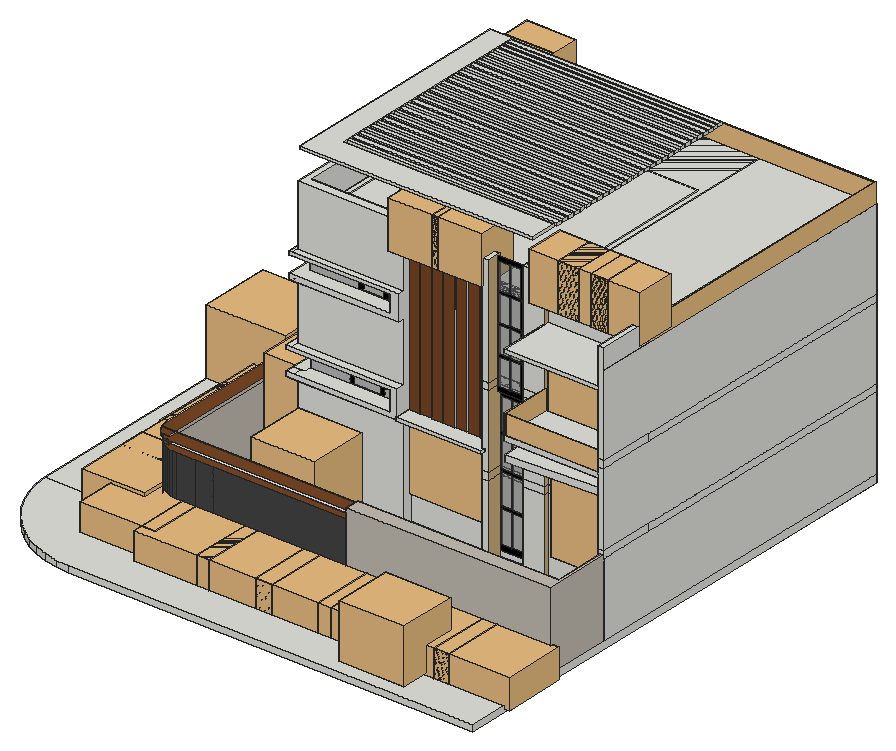
# SketchUp Ruby script. Lengths in inches.
U = 1.inch
M = Sketchup.active_model
def pt(a) = Geom::Point3d.new(a.map { |v| v * U })
def face(e, loops, mat)
  f = e.add_face(loops[0].map { |a| pt(a) })
  loops[1..].each { |l| e.add_face(l.map { |a| pt(a) }).erase! }
  f.material = f.back_material = mat if mat
  f
end
# faces: each face lists its corners as indices into pts; further lists are holes
def faces(e, pts, list, mat = nil) = list.each { |f| face(e, (f[0].is_a?(Array) ? f : [f]).map { |l| l.map { |i| pts[i] } }, mat) }
# xy, xz, yz: faces in a plane at the given z, y or x. An outline is a flat list of corners, or four numbers for a rectangle; further outlines are holes
def ring(l) = l.size == 4 ? [[l[0], l[1]], [l[2], l[1]], [l[2], l[3]], [l[0], l[3]]] : l.each_slice(2).to_a
def flat(e, list, mat, &to3) = list.each { |f| face(e, (f[0].is_a?(Array) ? f : [f]).map { |l| ring(l).map { |u, v| to3.(u, v) } }, mat) }
def xy(e, z, list, mat = nil) = flat(e, list, mat) { |x, y| [x, y, z] }
def xz(e, y, list, mat = nil) = flat(e, list, mat) { |x, z| [x, y, z] }
def yz(e, x, list, mat = nil) = flat(e, list, mat) { |y, z| [x, y, z] }
def lines(e, pts, list) = list.each { |a, b| e.add_line(pt(pts[a]), pt(pts[b])) }
# prism: a flat outline (further loops are holes) pulled along v
def prism(e, loops, v, mat = nil)
  f = face(e, loops, mat); d = Geom::Vector3d.new(v.map { |x| x * U })
  f.pushpull(f.normal.samedirection?(d) ? d.length : -d.length)
end
def box(e, o, s, mat = nil) = prism(e, [[o, [o[0] + s[0], o[1], o[2]], [o[0] + s[0], o[1] + s[1], o[2]], [o[0], o[1] + s[1], o[2]]]], [0, 0, s[2]], mat)
def at(x, y, z, deg = 0) = Geom::Transformation.translation(pt([x, y, z])) * Geom::Transformation.rotation(ORIGIN, Z_AXIS, deg.degrees)
def axes(o, x, y, z) = Geom::Transformation.new([*x, 0, *y, 0, *z, 0, *pt(o).to_a, 1])
def part(name) = M.definitions.add(name)
# library, detail: a bought-in or finely detailed component or shape, given as its bounding box
def library(name, o, s) = part(name).tap { |d| box(d.entities, o, s) }
def detail(e, o, s) = box(e.add_group.entities, o, s)
def put(e, d, t, mat = nil) = e.add_instance(d, t).tap { |i| i.material = mat if mat }
def group(e, t, mat = nil) = e.add_group.tap { |g| g.transformation = t; g.material = mat if mat }.entities
root = M.entities
M.materials.add("[Color D01]").color = [221, 214, 193]
M.materials.add("[Color M00]").color = [255, 255, 255]
M.materials.add("[Color M09]").color = [0, 0, 0]
M.materials.add("[Field Rectangle Tile]").color = [196, 189, 179]
M.materials.add("[Field Rectangle Tile]1").color = [196, 189, 179]
M.materials.add("[Granite Dark Gray]").color = [69, 68, 68]
M.materials.add("[Mirror 01]").color = [185, 185, 185]
M.materials.add("[Translucent_Glass_Gray]").color = [128, 128, 128]
M.materials["[Translucent_Glass_Gray]"].alpha = 0.5
M.materials.add("[Wood Floor Light]").color = [204, 176, 127]
M.materials.add("[Wood Floor]").color = [155, 105, 61]
M.materials.add("[Wood Veneer 01]").color = [120, 70, 37]
c1 = library("window full",[0,0,0],[14.17,66.54,74.02])
c2 = library("PENTEK_RP+Hermetic+70+FP_EI90_Single_Leaf_Door_Top__And_Both",[-0.01,-3.31,-0.39],[86.62,9.05,102.36])
c3 = library("Ver Glass Railing",[0,0,0],[2.5,185,31])
c4 = library("Glazed panel assembly",[0,0,0],[135.86,2.83,115.35])
c5 = part("wndow2")
xz(c5.entities,0,[[[-13,0,13,55],[-11,2,11,53]],[-0.5,2,0.5,2,0.5,14.25,11,14.25,11,15.25,0.5,15.25,0.5,27,11,27,11,28,0.5,28,0.5,39.75,11,39.75,11,40.75,0.5,40.75,0.5,53,-0.5,53,-0.5,40.75,-11,40.75,-11,39.75,-0.5,39.75,-0.5,28,-11,28,-11,27,-0.5,27,-0.5,15.25,-11,15.25,-11,14.25,-0.5,14.25]],"[Color M09]")
xz(c5.entities,0,[[-11,2,-0.5,14.25],[0.5,2,11,14.25],[-11,15.25,-0.5,27],[0.5,15.25,11,27],[-11,28,-0.5,39.75],
  [0.5,28,11,39.75],[-11,40.75,-0.5,53],[0.5,40.75,11,53]],"[Translucent_Glass_Gray]")
c6 = library("windows",[1167.36,374.41,0],[108.46,5.67,65.67])
c7 = library("Round Planter with Plant",[-35.48,-39.77,0],[80.62,63.55,77.875])
c8 = library("GoldenBamboo",[-21.19,-21.7,-0.46],[44.22,41.02,72.81])
c9 = library("Hedge section",[-5.85,-6.78,-4.2],[64.5,123.13,48])
c10 = library("279",[-34.23,-17.84,-5],[65.55,41.78,17.48])
c11 = library("Palm+in+pot",[-44.1,-44.03,0.04],[106.77,95.72,88.04])
c12 = library("ganyedes's+yellow&green+tree",[-30.91,-35.46,0],[63.51,67.02,85.79])
c13 = part("Group\#12")
box(c13.entities,[0,0,0],[344.0625,7.58,4.6875])
xy(root,-12,[[0,161.3125,168.75,829],[265.5625,346.4375,275.875,492.0625],[267.4375,748.89,275.875,808.39]])
xy(root,-10.75,[[275.875,346.4375,438.125,361.3125]])
xy(root,-2.125,[[168.75,0,829.125,0,829.125,161.3125,0,161.3125,2.76,140.16,8.11,119.5,15.95,99.66,26.17,80.9375,38.62,63.61,53.11,47.95,69.41,34.18,87.28,22.53,106.44,13.16,126.62,6.22,147.49,1.81],[0,161.3125,168.75,829]])
xy(root,-1.0625,[[239.8125,808.39,277.27,827.375]])
xy(root,0,[[491.9375,162.5,825.8125,162.5,825.8125,271.3125,819.83,271.3125,819.83,185.9375,491.9375,185.9375],[816.01,271.3125,816.01,361.3125,825.8125,361.3125,825.8125,271.4375,819.83,271.4375,819.83,271.3125],[819.83,271.3125,825.8125,271.4375],[[573.62,338.0625,573.62,361.3125,275.875,361.3125,275.875,827.375,825.8125,827.375,825.8125,361.3125,662.88,361.3125,662.88,353.3125,627,353.3125,627,361.3125,583.89,361.3125,583.89,338.0625],[284.875,370.3125,626.875,712.3125]],[284.875,370.3125,626.875,712.3125],
  [168.75,491.6875,168.75,829,175.75,829,175.75,821.49,195.4375,821.49,195.4375,491.6875],[267.4375,748.89,275.875,808.39],[175.75,821.49,239.8125,829]])
xy(root,0,[[214.63,162.5,208.88,162.86,203.22,163.94,197.73,165.72,192.52,168.17,187.65,171.25,185.98,172.625,194.0625,172.625,194.0625,179.125,491.9375,179.125,491.9375,162.5],[185.98,172.625,183.2,174.92,179.25,179.12,175.85,183.78,173.07,188.82,170.93,194.18,169.49,199.76,168.75,205.47,168.75,491.6875,180.875,491.6875,180.875,179.125,194.0625,179.125,194.0625,172.625]],"[Field Rectangle Tile]")
xy(root,108.91,[[214.63,162.5,491.9375,162.5,491.9375,179.125,194.0625,179.125,194.0625,172.625,185.98,172.625,187.65,171.25,192.52,168.17,197.73,165.72,203.22,163.94,208.88,162.86],[185.98,172.625,194.0625,172.625,194.0625,179.125,180.875,179.125,180.875,491.6875,168.75,491.6875,168.75,205.47,169.49,199.76,170.93,194.18,173.07,188.82,175.85,183.78,179.25,179.12,183.2,174.92]],"[Wood Veneer 01]")
xy(root,118.68,[[206.91,162.5,491.9375,162.5,491.9375,185.9375,195.4375,185.9375,195.4375,171.6875,182.2,171.6875,183.68,170.39,187.83,167.61,192.31,165.41,197.04,163.8,201.93,162.83],[182.2,171.6875,195.4375,171.6875,195.4375,185.9375,171.72,185.9375,173.86,181.58,176.64,177.43,179.93,173.68],[171.72,185.9375,195.4375,185.9375,195.4375,491.6875,168.75,491.6875,168.75,200.66,169.08,195.68,170.05,190.79,171.66,186.06]],"[Wood Veneer 01]")
xy(root,120,[[[816.01,271.3125,819.83,271.3125,819.83,271.4375,825.8125,271.4375,825.8125,827.375,275.875,827.375,275.875,808.39,267.4375,808.39,267.4375,748.89,275.875,748.89,275.875,361.3125,573.62,361.3125,573.62,338.0625,583.89,338.0625,583.89,361.3125,816.01,361.3125],[284.875,370.3125,626.875,712.3125]],[627,353.3125,662.88,361.3125]])
xy(root,120,[[819.83,271.3125,825.8125,271.4375]],"[Field Rectangle Tile]")
xy(root,121.96,[[206.91,162.5,201.93,162.83,197.04,163.8,192.31,165.41,187.83,167.61,183.68,170.39,182.2,171.6875,195.4375,171.6875,195.4375,185.9375,491.9375,185.9375,491.9375,162.5],[182.2,171.6875,179.93,173.68,176.64,177.43,173.86,181.58,171.72,185.9375,195.4375,185.9375,195.4375,171.6875],[171.72,185.9375,171.66,186.06,170.05,190.79,169.08,195.68,168.75,200.66,168.75,491.6875,195.4375,491.6875,195.4375,185.9375]],"[Wood Veneer 01]")
xy(root,124.03,[[175.75,821.49,239.8125,829]],"[Field Rectangle Tile]")
xy(root,125.47,[[491.9375,162.5,491.9375,185.9375,819.83,185.9375,819.83,271.3125,825.8125,271.3125,825.8125,162.5],[168.75,491.6875,195.4375,491.6875,195.4375,821.49,175.75,821.49,175.75,829,168.75,829]],"[Field Rectangle Tile]")
xy(root,132,[[[816.01,271.3125,816.01,361.3125,583.89,361.3125,583.89,338.0625,573.62,338.0625,573.62,361.3125,275.875,361.3125,275.875,748.89,267.4375,748.89,267.4375,808.39,277.27,808.39,277.27,827.375,825.8125,827.375,825.8125,271.3125],[284.875,370.3125,626.875,712.3125]],[627,353.3125,662.88,361.3125],[284.875,370.3125,626.875,712.3125]])
xy(root,160.08,[[438.125,330.8125,438.125,361.3125,573.62,361.3125,573.62,338.0625,577.3125,338.0625,577.3125,330.8125],[573.62,338.0625,577.3125,361.3125]])
xy(root,160.1,[[255.6875,333.625,265.5625,492.0625],[265.5625,333.625,438.125,346.4375]])
xy(root,165.14,[[438.125,330.8125,577.3125,330.8125,577.3125,338.0625,573.62,338.0625,573.62,361.3125,455.875,361.3125,455.875,357.1875,438.125,357.1875],[573.62,338.0625,577.3125,361.3125]])
xy(root,167.29,[[255.6875,333.625,268.5625,349.4375],[268.5625,333.625,425.75,333.625,425.75,361.0625,275.875,361.0625,275.875,349.4375,268.5625,349.4375],[255.6875,349.4375,275.875,478]])
xy(root,199.99,[[255.6875,333.625,268.5625,349.4375],[268.5625,333.625,268.5625,349.4375,275.875,349.4375,275.875,361.0625,425.75,361.0625,425.75,333.625],[255.6875,349.4375,275.875,478]])
xy(root,206.11,[[255.6875,333.625,265.5625,492.0625],[265.5625,333.625,438.125,346.4375]])
xy(root,207.82,[[667.38,267.22,662.88,353.3125,816.01,361.3125,820.5,275.22]])
xy(root,218.69,[[667.38,267.22,820.5,275.22,816.01,361.3125,662.88,353.3125]])
xy(root,225.91,[[223.8125,591.58,275.875,748.89]])
xy(root,232.53,[[223.8125,591.58,275.875,748.89]])
xy(root,235.77,[[662.88,271.3125,816.01,361.3125]])
xy(root,245,[[662.88,271.3125,816.01,361.3125]])
xy(root,252,[[[816.01,271.3125,825.8125,271.3125,825.8125,827.375,239.8125,827.375,239.8125,808.39,267.4375,808.39,267.4375,748.89,275.875,748.89,275.875,361.3125,573.62,361.3125,573.62,338.0625,583.89,338.0625,583.89,361.3125,627,361.3125,627,353.3125,662.88,353.3125,662.88,361.3125,816.01,361.3125],[284.875,370.3125,626.875,712.3125]],[223.8125,591.58,275.875,740.64],[223.8125,740.64,275.875,748.89]])
xy(root,258.25,[[223.8125,601.46,275.875,740.64]])
xy(root,264,[[573.62,337.875,583.89,338.0625],[284.875,370.3125,626.875,712.3125]])
xy(root,302.1875,[[265.5625,336.5625,438.125,346.4375]])
xy(root,302.3,[[259.1875,336.5625,265.5625,492.0625]])
xy(root,310.68,[[259.1875,336.5625,423.3125,336.5625,423.3125,360,274.875,360,274.875,476.5,259.1875,476.5]])
xy(root,337.87,[[268.5625,336.5625,268.5625,349.4375,274.875,349.4375,274.875,360,423.3125,360,423.3125,336.5625]])
xy(root,337.99,[[259.1875,336.5625,259.1875,476.5,274.875,476.5,274.875,349.4375,268.5625,349.4375,268.5625,336.5625]])
xy(root,338.02,[[253.0625,498.98,275.875,565.79]])
xy(root,340.52,[[253.0625,498.98,275.875,565.79]])
xy(root,343.56,[[259.1875,336.5625,265.5625,492.0625],[265.5625,336.5625,438.125,346.4375]])
xy(root,361.8125,[[223.8125,601.46,275.875,740.64]])
xy(root,364.17,[[662.88,271.3125,816.01,361.3125]])
xy(root,369.65,[[662.88,271.3125,816.01,361.3125]])
xy(root,369.9375,[[223.8125,591.58,275.875,743.08],[223.8125,743.08,275.875,748.89]])
xy(root,396,[[825.23,271.3125,825.8125,271.3125,825.8125,827.375,275.875,827.375,275.875,566.29,284.875,566.29,284.875,712.3125,626.875,712.3125,626.875,370.3125,284.875,370.3125,284.875,492.0625,275.875,492.0625,275.875,361.3125,825.23,361.3125],[438.125,357.1875,455.875,361.3125],[457.4375,357.1875,475.1875,361.3125],[476.6875,357.1875,494.4375,361.3125],[496.0625,357.1875,513.8125,361.3125],
  [516.0625,357.1875,533.8125,361.3125],[536.3125,357.1875,554.0625,361.3125],[555.87,357.1875,573.62,361.3125],[409.12,375.75,426.56,383.06],[291.63,576.24,309.26,602.43],
  [293.42,673.58,312.92,704.71]])
xy(root,426.5625,[[275.875,492.0625,284.875,566.29]])
xy(root,428.375,[[816.01,271.3125,825.23,361.3125]])
xy(root,432.4375,[[267.4375,748.89,275.875,827.375],[239.8125,808.39,267.4375,827.375]])
xy(root,443.3125,[[573.62,337.875,583.89,361.3125],[265.5625,346.4375,438.125,346.4375,438.125,361.3125,275.875,361.3125,275.875,492.0625,265.5625,492.0625],[627,353.3125,662.88,361.3125]])
xy(root,493.6875,[[271.05,344.17,271.05,732.64,293.42,732.64,293.42,602.43,291.63,602.43,291.63,576.24,293.42,576.24,293.42,344.17],[293.42,344.17,293.42,576.24,308.57,576.24,308.57,386.78,312.92,386.78,312.92,344.17],[312.92,344.17,312.92,386.78,409.12,386.78,409.12,375.75,426.56,375.75,426.56,386.78,651.74,386.78,651.74,344.17],[409.12,375.75,426.56,383.06],[409.12,383.06,426.56,386.78],
  [291.63,576.24,293.42,602.43],[293.42,576.24,308.57,602.43],[308.57,576.24,309.26,602.43],[293.42,602.43,308.57,673.58],[308.57,673.58,312.92,704.71],
  [293.42,704.71,308.57,732.64]])
xy(root,498.375,[[271.05,344.17,651.74,344.17,651.74,386.78,308.57,386.78,308.57,732.64,271.05,732.64]])
xz(root,0,[[168.75,-12,829.125,-2.125]])
xz(root,161.3125,[[168.75,-12,829.125,-2.125]])
xz(root,162.5,[[206.91,118.68,491.9375,121.96]],"[Color M00]")
xz(root,162.5,[[491.9375,0,825.8125,125.47]],"[Field Rectangle Tile]1")
xz(root,162.5,[[214.63,0,245.35,108.91],[245.35,0,273.69,108.91],[273.69,0,491.9375,108.91]],"[Granite Dark Gray]")
xz(root,171.6875,[[182.2,118.68,195.4375,121.96]],"[Wood Veneer 01]")
xz(root,179.125,[[180.875,0,491.9375,108.91]],"[Field Rectangle Tile]")
xz(root,185.9375,[[491.9375,0,819.83,0,819.83,125.47,491.9375,125.47,491.9375,121.96,171.72,121.96,171.72,118.68,491.9375,118.68]],"[Field Rectangle Tile]")
xz(root,271.3125,[[816.01,0,825.8125,120],[816.01,120,819.83,120,819.83,125.47,825.8125,125.47,825.8125,132,816.01,132],[816.01,132,825.8125,252],[662.88,235.77,816.01,245],[816.01,252,825.8125,264],
  [816.01,264,825.8125,264,825.8125,396,825.23,396,825.23,428.375,816.01,428.375],[662.88,364.17,816.01,369.65]])
xz(root,271.3125,[[819.83,120,825.8125,125.47]],"[Field Rectangle Tile]")
xz(root,271.4375,[[819.83,0,825.8125,120]])
xz(root,330.8125,[[438.125,160.08,577.3125,165.14]])
xz(root,333.625,[[255.6875,160.1,438.125,160.1,438.125,206.11,255.6875,206.11,255.6875,199.99,425.75,199.99,425.75,167.29,255.6875,167.29]])
xz(root,336.5625,[[265.5625,302.1875,438.125,302.1875,438.125,343.56,259.1875,343.56,259.1875,337.99,268.5625,337.99,268.5625,337.87,423.3125,337.87,423.3125,310.68,259.1875,310.68,259.1875,302.3,265.5625,302.3]])
xz(root,337.875,[[573.62,264,583.89,443.3125]])
xz(root,338.0625,[[573.62,0,583.89,120],[573.62,120,583.89,132],[573.62,132,583.89,132,583.89,252,573.62,252,573.62,165.14,577.3125,165.14,577.3125,160.08,573.62,160.08],[573.62,252,583.89,264]])
xz(root,344.17,[[271.05,493.6875,651.74,498.375]])
xz(root,346.4375,[[265.5625,-12,275.875,-12,275.875,-10.75,438.125,-10.75,438.125,160.1,265.5625,160.1],[265.5625,206.11,438.125,302.1875],[268.5625,305.1875,268.5625,305.3,265.5625,305.3],[265.5625,343.56,438.125,443.3125]])
xz(root,349.4375,[[268.5625,337.87,274.875,337.99]])
xz(root,353.3125,[[627,0,662.88,120],[627,120,662.88,132],[627,132,662.88,252],[627,252,662.88,264],[627,264,662.88,443.3125]])
xz(root,357.1875,[[438.125,165.14,455.875,396],[457.4375,165.14,475.1875,396],[476.6875,165.14,494.4375,396],[496.0625,165.14,513.8125,396],[516.0625,165.14,533.8125,396],
  [536.3125,165.14,554.0625,396],[555.87,165.14,573.62,396]],"[Wood Veneer 01]")
xz(root,360,[[355,310.68,362.92,337.87],[362.92,310.68,394.76,311.6],[394.76,310.68,401.17,335.18],[362.92,335.18,401.17,337.87]],"[Color M09]")
xz(root,360,[[274.875,310.68,355,337.87],[401.17,310.68,423.3125,337.87],[362.92,311.6,394.76,335.18]],"[Mirror 01]")
xz(root,361.0625,[[338.0625,167.29,347,199.99],[347,167.29,388.17,168.73],[388.17,167.29,395.3125,197.49],[347,197.49,395.3125,199.99]],"[Color M09]")
xz(root,361.0625,[[275.875,167.29,338.0625,199.99],[395.3125,167.29,425.75,199.99],[347,168.73,388.17,197.49]],"[Mirror 01]")
xz(root,361.3125,[[816.01,-12,825.8125,0],[275.875,-10.75,438.125,0],[275.875,0,438.125,120],[438.125,0,573.62,120],[583.89,0,627,120],
  [662.88,0,816.01,120],[275.875,120,438.125,132],[438.125,120,573.62,132],[583.89,120,627,132],[627,120,662.88,132],
  [662.88,120,816.01,132],[275.875,132,438.125,252],[438.125,132,573.62,160.08],[583.89,132,627,252],[662.88,132,816.01,235.77],
  [438.125,160.08,573.62,165.14],[573.62,160.08,577.3125,165.14],[438.125,165.14,455.875,252],[455.875,165.14,475.1875,252],[475.1875,165.14,494.4375,252],
  [494.4375,165.14,513,252],[513,165.14,513.31,252,513,252],[513,165.14,533.8125,165.14,533.8125,252,513.31,252],[533.8125,165.14,553.25,252],[553.25,165.14,553.25,252,553.56,252],
  [553.25,165.14,569.93,165.14,569.93,252,553.56,252],[569.93,165.14,573.62,252],[662.88,245,816.01,252],[275.875,252,438.125,264],[455.875,252,475.1875,264],
  [475.1875,252,494.4375,264],[494.4375,252,513,252,513.32,256.76,513.35,264,494.4375,264],[513,252,513.31,252,513.32,256.76,513.35,264,513.8125,264,513.32,256.76],[513,252,513.31,252,513.32,256.76],[513.31,252,533.8125,252,533.8125,264,513.8125,264,513.32,256.76],
  [533.8125,252,553.25,252,553.57,256.76,553.6,264,533.8125,264],[553.25,252,553.56,252,553.57,256.76,553.6,264,554.0625,264,553.57,256.76],[553.25,252,553.56,252,553.57,256.76],[553.56,252,569.93,252,569.93,264,554.0625,264,553.57,256.76],[569.93,252,573.62,264],
  [583.89,252,627,264],[662.88,252,816.01,264],[275.875,264,438.125,396],[455.875,264,475.1875,396],[475.1875,264,494.4375,396],
  [494.4375,264,513.35,264,513.8125,396,494.4375,396],[513.35,264,513.8125,396,513.8125,264],[513.8125,264,533.8125,396],[533.8125,264,553.6,264,554.0625,396,533.8125,396],[553.6,264,554.0625,264,554.0625,396],
  [554.0625,264,569.93,396],[569.93,264,573.62,396],[583.89,264,627,396],[662.88,264,816.01,364.17],[662.88,369.65,816.01,396],
  [275.875,396,438.125,443.3125],[573.62,396,583.89,443.3125],[627,396,662.88,443.3125],[816.01,396,825.23,428.375]])
xz(root,370.3125,[[284.875,0,626.875,120],[284.875,132,626.875,252],[284.875,264,626.875,396]])
xz(root,375.75,[[409.12,396,426.56,493.6875]])
xz(root,383.06,[[409.12,396,426.56,493.6875]])
xz(root,386.78,[[308.57,493.6875,651.74,498.375]])
xz(root,476.5,[[259.1875,310.68,274.875,337.99]])
xz(root,478,[[255.6875,167.29,275.875,199.99]])
xz(root,491.6875,[[168.75,0,180.875,108.91],[180.875,0,195.4375,108.91]],"[Field Rectangle Tile]")
xz(root,491.6875,[[168.75,108.91,195.4375,118.68],[168.75,121.96,195.4375,125.47]],"[Wood Veneer 01]")
xz(root,492.0625,[[265.5625,-12,265.5625,160.1,255.6875,160.1,255.6875,206.11,265.5625,206.11,265.5625,302.3,259.1875,302.3,259.1875,343.56,265.5625,343.56,265.5625,443.3125,275.875,443.3125,275.875,-12],[275.875,396,284.875,426.5625]])
xz(root,498.98,[[253.0625,338.02,275.875,340.52]])
xz(root,565.79,[[253.0625,338.02,275.875,340.52]])
xz(root,566.29,[[275.875,396,284.875,426.5625]])
xz(root,576.24,[[291.63,396,309.26,493.6875]])
xz(root,591.58,[[223.8125,225.91,275.875,232.53],[223.8125,252,275.875,369.9375]])
xz(root,601.46,[[223.8125,258.25,275.875,361.8125]])
xz(root,602.43,[[291.63,396,309.26,493.6875]])
xz(root,673.58,[[293.42,396,312.92,493.6875]])
xz(root,704.71,[[293.42,396,312.92,493.6875]])
xz(root,712.3125,[[284.875,0,626.875,120],[284.875,132,626.875,252],[284.875,264,626.875,396]])
xz(root,732.64,[[271.05,493.6875,308.57,498.375]])
xz(root,740.64,[[223.8125,258.25,275.875,361.8125]])
xz(root,748.89,[[267.4375,-12,275.875,0],[223.8125,225.91,267.4375,232.53],[223.8125,252,267.4375,369.9375]])
xz(root,748.89,[[267.4375,0,275.875,120],[267.4375,120,275.875,132],[267.4375,132,275.875,225.91],[267.4375,232.53,275.875,252],[267.4375,369.9375,275.875,432.4375]],"[Wood Floor]")
xz(root,808.39,[[267.4375,-12,275.875,-1.0625],[267.4375,-1.0625,275.875,0],[275.875,-1.0625,277.27,-1.0625,277.27,132,267.4375,132,267.4375,120,275.875,120],[267.4375,0,275.875,120]])
xz(root,808.39,[[239.8125,-1.0625,267.4375,252],[239.8125,252,267.4375,264],[239.8125,264,267.4375,367.5625],[239.8125,367.5625,267.4375,369.9375],[239.8125,369.9375,267.4375,432.4375]],"[Color D01]")
xz(root,821.49,[[175.75,0,195.4375,124.03],[195.4375,0,239.8125,124.03],[175.75,124.03,195.4375,125.47]],"[Field Rectangle Tile]")
xz(root,827.375,[[239.8125,-1.0625,239.8125,252,825.8125,252,825.8125,132,277.27,132,277.27,120,275.875,120,275.875,0,277.27,0,277.27,-1.0625],[275.875,0,277.27,120],[277.27,0,825.8125,120],[239.8125,252,275.875,264],[239.8125,264,239.8125,432.4375,275.875,432.4375,275.875,396,825.8125,396,825.8125,264]])
xz(root,829,[[0,-12,168.75,-2.125]])
xz(root,829,[[168.75,0,175.75,125.47],[175.75,0,239.8125,124.03]],"[Field Rectangle Tile]")
yz(root,0,[[161.3125,-12,829,-2.125]])
yz(root,168.75,[[161.3125,-12,829,-2.125]])
yz(root,168.75,[[200.66,118.68,491.6875,121.96]],"[Color M00]")
yz(root,168.75,[[491.6875,0,829,125.47]],"[Field Rectangle Tile]1")
yz(root,168.75,[[205.47,0,236.51,108.91],[236.51,0,266.86,108.91],[266.86,0,491.6875,108.91]],"[Granite Dark Gray]")
yz(root,175.75,[[821.49,0,829,124.03],[821.49,124.03,829,125.47]])
yz(root,180.875,[[179.125,0,491.6875,108.91]],"[Field Rectangle Tile]")
yz(root,195.4375,[[491.6875,0,821.49,0,821.49,125.47,491.6875,125.47,491.6875,121.96,171.6875,121.96,171.6875,118.68,491.6875,118.68]],"[Field Rectangle Tile]")
yz(root,223.8125,[[591.58,225.91,748.89,232.53],[591.58,252,591.58,369.9375,743.08,369.9375,743.08,361.8125,601.46,361.8125,601.46,258.25,740.64,258.25,740.64,252],[740.64,252,740.64,361.8125,743.08,361.8125,743.08,369.9375,748.89,369.9375,748.89,252]])
yz(root,239.8125,[[821.49,0,827.375,124.03],[827.375,0,829,124.03]])
yz(root,239.8125,[[808.39,-1.0625,808.39,252,827.375,252,827.375,124.03,821.49,124.03,821.49,0,827.375,0,827.375,-1.0625],[808.39,252,827.375,264],[808.39,264,827.375,367.5625],[808.39,367.5625,827.375,369.9375],[808.39,369.9375,827.375,432.4375]],"[Color D01]")
yz(root,253.0625,[[498.98,338.02,565.79,340.52]])
yz(root,255.6875,[[333.625,160.1,333.625,167.29,478,167.29,478,199.99,333.625,199.99,333.625,206.11,492.0625,206.11,492.0625,160.1]])
yz(root,259.1875,[[336.5625,302.3,336.5625,310.68,476.5,310.68,476.5,337.99,336.5625,337.99,336.5625,343.56,492.0625,343.56,492.0625,302.3]])
yz(root,265.5625,[[346.4375,-12,492.0625,160.1],[346.4375,206.11,346.4375,302.1875,336.5625,302.1875,336.5625,302.3,492.0625,302.3,492.0625,206.11],[346.4375,343.56,492.0625,443.3125]])
yz(root,267.4375,[[748.89,-12,808.39,0]])
yz(root,267.4375,[[748.89,0,808.39,120],[748.89,120,808.39,132],[748.89,132,808.39,252],[748.89,252,808.39,264],[748.89,264,808.39,367.5625],
  [748.89,367.5625,808.39,369.9375],[748.89,369.9375,808.39,432.4375]],"[Wood Floor]")
yz(root,268.5625,[[336.5625,305.1875,346.4375,305.3],[336.5625,337.87,349.4375,337.99]])
yz(root,271.05,[[344.17,493.6875,732.64,498.375]])
yz(root,274.875,[[349.4375,337.87,360,337.99]])
yz(root,274.875,[[424.53,310.68,433.53,337.99]],"[Color M09]")
yz(root,274.875,[[360,310.68,424.53,337.99],[433.53,310.68,476.5,337.99]],"[Mirror 01]")
yz(root,275.875,[[346.4375,-12,361.3125,-10.75],[361.3125,-12,492.0625,0],[748.89,-12,808.39,0],[361.3125,0,492.0625,120],[808.39,0,827.375,120],
  [361.3125,120,492.0625,132],[361.3125,132,361.3125,167.29,478,167.29,478,199.99,361.3125,199.99,361.3125,252,492.0625,252,492.0625,132],[361.0625,167.29,361.3125,199.99],[361.3125,252,492.0625,264],[591.58,252,591.58,363.25,626.21,363.25,626.21,361.8125,601.46,361.8125,601.46,258.25,740.64,258.25,740.64,252],
  [601.46,258.25,732.96,264],[732.96,258.25,740.64,264],[361.3125,264,492.0625,396],[601.46,264,740.64,361.8125],[591.58,363.25,591.58,369.9375,625.14,369.9375,625.14,367.5625,626.21,367.5625,626.21,363.25],
  [361.3125,396,492.0625,443.3125],[748.89,396,827.375,432.4375]])
yz(root,275.875,[[492.0625,0,748.89,120],[492.0625,120,748.89,132],[492.0625,132,492.0625,252,748.89,252,748.89,232.53,591.58,232.53,591.58,225.91,748.89,225.91,748.89,132],[492.0625,252,591.58,264],[[492.0625,264,492.0625,426.5625,566.29,426.5625,566.29,396,748.89,396,748.89,369.9375,591.58,369.9375,591.58,264],[498.98,338.02,565.79,340.52]]],"[Color D01]")
yz(root,275.875,[[425.1875,167.29,435.35,199.99]],"[Color M09]")
yz(root,275.875,[[361.3125,167.29,425.1875,199.99],[435.35,167.29,478,199.99]],"[Mirror 01]")
yz(root,277.27,[[808.39,-1.0625,827.375,132]])
yz(root,284.875,[[370.3125,0,712.3125,120],[370.3125,132,712.3125,252],[370.3125,264,712.3125,264,712.3125,396,566.29,396,566.29,426.5625,492.0625,426.5625,492.0625,396,370.3125,396]])
yz(root,291.63,[[576.24,396,602.43,493.6875]])
yz(root,293.42,[[673.58,396,704.71,493.6875]])
yz(root,308.57,[[386.78,493.6875,391.91,498.375],[399.5,493.6875,732.64,498.375]])
yz(root,309.26,[[576.24,396,602.43,493.6875]])
yz(root,312.92,[[673.58,396,704.71,493.6875]])
yz(root,409.12,[[375.75,396,383.06,493.6875]])
yz(root,423.3125,[[336.5625,310.68,360,337.87]])
yz(root,425.75,[[333.625,167.29,361.0625,199.99]])
yz(root,426.56,[[375.75,396,383.06,493.6875]])
yz(root,438.125,[[346.4375,-10.75,361.3125,160.08],[330.8125,160.08,330.8125,165.14,333.625,165.14,333.625,160.1,346.4375,160.1,346.4375,160.08],[346.4375,160.08,361.3125,160.08,361.3125,165.14,333.625,165.14,333.625,160.1,346.4375,160.1],[333.625,165.14,357.1875,165.14,357.1875,443.3125,346.4375,443.3125,346.4375,343.56,336.5625,343.56,336.5625,302.1875,346.4375,302.1875,346.4375,206.11,333.625,206.11],[357.1875,165.14,361.3125,396],
  [357.1875,396,361.3125,443.3125]])
yz(root,455.875,[[357.1875,165.14,361.3125,396]])
yz(root,475.1875,[[357.1875,165.14,361.3125,396]])
yz(root,491.9375,[[162.5,0,179.125,108.91],[179.125,0,185.9375,108.91]],"[Field Rectangle Tile]")
yz(root,491.9375,[[162.5,108.91,185.9375,118.68],[162.5,121.96,185.9375,125.47]],"[Wood Veneer 01]")
yz(root,494.4375,[[357.1875,165.14,361.3125,396]])
yz(root,533.8125,[[357.1875,165.14,361.3125,396]])
yz(root,573.62,[[338.0625,0,361.3125,120],[338.0625,120,361.3125,132],[338.0625,132,361.3125,160.08],[338.0625,165.14,357.1875,252],[357.1875,165.14,361.3125,252],
  [338.0625,252,357.1875,264],[357.1875,252,361.3125,264],[337.875,264,357.1875,443.3125],[357.1875,264,361.3125,396],[357.1875,396,361.3125,443.3125]])
yz(root,577.3125,[[330.8125,160.08,338.0625,165.14],[338.0625,160.08,361.3125,165.14]])
yz(root,583.89,[[338.0625,0,361.3125,120],[338.0625,120,361.3125,132],[338.0625,132,361.3125,252],[338.0625,252,361.3125,264],[337.875,264,361.3125,443.3125]],"[Wood Floor Light]")
yz(root,626.875,[[370.3125,0,712.3125,120],[370.3125,132,712.3125,252],[370.3125,264,712.3125,396]])
yz(root,627,[[353.3125,0,361.3125,120],[353.3125,120,361.3125,132],[353.3125,132,361.3125,252]])
yz(root,627,[[353.3125,252,361.3125,264],[353.3125,264,361.3125,443.3125]],"[Wood Floor Light]")
yz(root,651.74,[[344.17,493.6875,386.78,498.375]])
yz(root,662.88,[[271.3125,235.77,353.3125,245],[271.3125,364.17,353.3125,369.65]])
yz(root,662.88,[[353.3125,0,361.3125,120],[353.3125,120,361.3125,132],[353.3125,132,361.3125,235.77],[353.3125,245,361.3125,252],[353.3125,252,361.3125,264],
  [353.3125,264,361.3125,364.17],[353.3125,369.65,361.3125,443.3125]],"[Wood Floor Light]")
yz(root,816.01,[[271.3125,0,361.3125,120],[271.3125,120,361.3125,132],[271.3125,132,361.3125,235.77],[271.3125,245,361.3125,252],[271.3125,252,361.3125,264],
  [271.3125,264,361.3125,364.17],[271.3125,369.65,361.3125,428.375]])
yz(root,819.83,[[185.9375,0,271.4375,0,271.4375,120,271.3125,120,271.3125,125.47,185.9375,125.47]],"[Field Rectangle Tile]")
yz(root,825.23,[[271.3125,396,361.3125,428.375]])
yz(root,825.8125,[[271.3125,0,271.4375,120],[271.4375,0,827.375,120],[271.3125,120,361.3125,132],[271.3125,132,827.375,252],[271.3125,252,361.3125,264],
  [271.3125,264,827.375,396]])
yz(root,825.8125,[[162.5,0,271.3125,125.47]],"[Field Rectangle Tile]")
yz(root,829.125,[[0,-12,161.3125,-2.125]])
p = [[147.49,1.81,-12],[168.75,0,-12],[168.75,0,-2.125],[147.49,1.81,-2.125],[126.62,6.22,-12],[126.62,6.22,-2.125],
  [106.44,13.16,-12],[106.44,13.16,-2.125],[87.28,22.53,-12],[87.28,22.53,-2.125],[69.41,34.18,-12],[69.41,34.18,-2.125],
  [53.11,47.95,-12],[53.11,47.95,-2.125],[38.62,63.61,-12],[38.62,63.61,-2.125],[26.17,80.9375,-12],[26.17,80.9375,-2.125],
  [15.95,99.66,-12],[15.95,99.66,-2.125],[8.11,119.5,-12],[8.11,119.5,-2.125],[2.76,140.16,-12],[2.76,140.16,-2.125],
  [0,161.3125,-12],[0,161.3125,-2.125],[214.63,162.5,108.91],[208.88,162.86,108.91],[208.88,162.86,0],[214.63,162.5,0],
  [203.22,163.94,108.91],[203.22,163.94,0],[197.73,165.72,108.91],[197.73,165.72,0],[192.52,168.17,108.91],[192.52,168.17,0],
  [187.65,171.25,108.91],[187.65,171.25,0],[185.98,172.625,108.91],[185.98,172.625,0],[183.2,174.92,108.91],[183.2,174.92,0],
  [179.25,179.12,108.91],[179.25,179.12,0],[175.85,183.78,108.91],[175.85,183.78,0],[173.07,188.82,108.91],[173.07,188.82,0],
  [170.93,194.18,108.91],[170.93,194.18,0],[169.49,199.76,108.91],[169.49,199.76,0],[168.75,205.47,108.91],[168.75,205.47,0],
  [201.93,162.83,121.96],[206.91,162.5,121.96],[206.91,162.5,118.68],[201.93,162.83,118.68],[197.04,163.8,121.96],[197.04,163.8,118.68],
  [192.31,165.41,121.96],[192.31,165.41,118.68],[187.83,167.61,121.96],[187.83,167.61,118.68],[183.68,170.39,121.96],[183.68,170.39,118.68],
  [182.2,171.6875,121.96],[182.2,171.6875,118.68],[179.93,173.68,121.96],[179.93,173.68,118.68],[176.64,177.43,121.96],[176.64,177.43,118.68],
  [173.86,181.58,121.96],[173.86,181.58,118.68],[171.72,185.9375,121.96],[171.72,185.9375,118.68],[171.66,186.06,121.96],[171.66,186.06,118.68],
  [170.05,190.79,121.96],[170.05,190.79,118.68],[169.08,195.68,121.96],[169.08,195.68,118.68],[168.75,200.66,121.96],[168.75,200.66,118.68],
  [513.8125,357.1875,165.14],[513,361.3125,165.14],[513.8125,357.1875,396],[513.8125,361.3125,396],[513.31,361.3125,252],[513.32,361.3125,256.76],
  [513.35,361.3125,264],[554.0625,357.1875,165.14],[553.25,361.3125,165.14],[554.0625,357.1875,396],[554.0625,361.3125,396],[553.56,361.3125,252],
  [553.57,361.3125,256.76],[553.6,361.3125,264],[662.88,353.3125,218.69],[662.88,353.3125,207.82],[667.38,267.22,207.82],[667.38,267.22,218.69],
  [820.5,275.22,218.69],[820.5,275.22,207.82],[816.01,361.3125,207.82],[816.01,361.3125,218.69],[268.5625,346.4375,305.1875],[265.5625,346.4375,305.3],
  [265.5625,349.4375,305.3],[265.5625,336.5625,305.3]]
faces(root,p,[[0,1,2,3],[4,0,3,5],[6,4,5,7],[8,6,7,9],[10,8,9,11],[12,10,11,13],[14,12,13,15],[16,14,15,17],
  [18,16,17,19],[20,18,19,21],[22,20,21,23],[24,22,23,25],[84,85,86],[87,86,85,88,89,90],[91,92,93],[94,93,92,95,96,97],
  [98,99,100,101],[102,101,100,103],[104,105,102,103],[98,105,104,99],[106,107,108]])
faces(root,p,[[26,27,28,29],[27,30,31,28],[30,32,33,31],[32,34,35,33],[34,36,37,35],[36,38,39,37],[38,40,41,39],[40,42,43,41],
  [42,44,45,43],[44,46,47,45],[46,48,49,47],[48,50,51,49],[50,52,53,51]],"[Granite Dark Gray]")
faces(root,p,[[54,55,56,57],[58,54,57,59],[60,58,59,61],[62,60,61,63],[64,62,63,65],[66,64,65,67],[68,66,67,69],[70,68,69,71],
  [72,70,71,73],[74,72,73,75],[76,74,75,77],[78,76,77,79],[80,78,79,81],[82,80,81,83]],"[Wood Veneer 01]")
lines(root,p,[[107,109]])
put(root,c1,at(269.6875,499.26,264))
put(root,c2,axes([270.61,739.29,260.79],[0,-1.19,0],[1,0,0],[0,0,1]))
put(root,c3,axes([223.8125,601.46,258.25],[1,0,0],[0,0.75234,0],[0,0,1]))
put(root,c2,axes([271.62,746.13,134.14],[0,-1.785,0],[0.74023,0,0],[0,0,0.9]))
put(root,c4,at(436.67,356.4375,42.76))
put(root,c5,axes([604.95,355.4375,244.04],[1.62,0,0],[0,1,0],[0,0,3.62322]))
put(root,c5,axes([604.95,360.69,9.25],[1.62,0,0],[0,1,0],[0,0,4.26116]))
put(root,c4,at(671.52,349.3125,249.05))
put(root,c3,axes([662.88,271.3125,245],[1,0,0],[0,0.44388,0],[0,0,1]))
put(root,c3,axes([665.6875,273.3125,245],[0,-1,0],[0.81253,0,0],[0,0,1]))
put(root,c6,axes([-536.7,-40.08,37.17],[1.04,0,0],[0,1.04,0],[0,0,2.4544]))
put(root,c3,axes([275.875,566.29,394],[3.11,0,0],[0,0.95152,0],[0,0,1]))
put(root,c3,axes([662.88,363.3125,396],[0,-1,0],[0.87753,0,0],[0,0,1]))
put(root,c3,axes([438.125,359.1875,396],[0,-1,0],[0.73713,0,0],[0,0,1]))
put(root,c3,axes([822.73,363.3125,396],[1,0,0],[0,2.50845,0],[0,0,1]))
put(root,c3,axes([275.875,827.375,396],[0,-1,0],[2.96947,0,0],[0,0,1]))
put(root,c7,at(301.73,654.73,396))
put(root,c7,at(301.73,789.36,396))
put(root,c7,at(301.73,743.92,396))
put(root,c7,at(301.73,615.29,396))
put(root,c7,at(682.02,382.25,401.07))
put(root,c7,at(729.52,382.25,401.07))
put(root,c7,at(782.58,382.25,401.07))
put(root,c8,axes([245.35,416.0625,-11.38],[2.35,0,0],[0,2.35,0],[0,0,2.35]))
put(root,c8,axes([332.86,280.46,-43.14],[2.35,0,0],[0,2.35,0],[0,0,2.35]))
put(root,c9,axes([130.07,171.57,-2.125],[0,-1.58,0],[1,0,0],[0,0,1]))
put(root,c9,axes([230.91,156.02,-2.125],[0,-1.58,0],[1,0,0],[0,0,1]))
put(root,c9,axes([333.41,156.02,-2.125],[0,-1.58,0],[1,0,0],[0,0,1]))
put(root,c9,axes([429.54,156.02,-2.125],[0,-1.58,0],[1,0,0],[0,0,1]))
put(root,c9,axes([169.64,257.9375,2.08],[-1.58,0,0],[0,-1,0],[0,0,1]))
put(root,c9,axes([169.64,339.25,2.08],[-1.58,0,0],[0,-1,0],[0,0,1]))
put(root,c9,axes([169.64,425.5,2.08],[-1.58,0,0],[0,-1,0],[0,0,1]))
put(root,c10,axes([70.05,401.94,2.7],[0,-1.82,0],[1.6,0,0],[0,0,1]))
put(root,c11,at(638.11,63.69,0))
put(root,c11,axes([52.87,545.37,-2.125],[1.22,0,0],[0,1.22,0],[0,0,1.22]))
put(root,c9,axes([169.64,530.25,2.08],[-1.58,0,0],[0,-1,0],[0,0,1]))
put(root,c9,axes([169.64,634.9375,2.08],[-1.58,0,0],[0,-1,0],[0,0,1]))
put(root,c9,axes([169.64,731,2.08],[-1.58,0,0],[0,-1,0],[0,0,1]))
put(root,c9,axes([169.64,828.375,2.08],[-1.58,0,0],[0,-1,0],[0,0,1]))
put(root,c9,axes([531.97,156.02,-2.125],[0,-1.58,0],[1,0,0],[0,0,1]))
put(root,c9,axes([621.91,156.02,-2.125],[0,-1.58,0],[1,0,0],[0,0,1]))
put(root,c9,axes([721.22,156.02,-2.125],[0,-1.58,0],[1,0,0],[0,0,1]))
put(root,c10,axes([70.05,763.18,2.7],[0,-1.82,0],[1.6,0,0],[0,0,1]))
put(root,c10,axes([70.05,652.74,2.7],[0,-1.82,0],[1.6,0,0],[0,0,1]))
put(root,c7,at(457.26,375.38,401.07))
put(root,c7,at(529.45,375.38,401.07))
put(root,c12,axes([246.67,708.28,0],[2.5239,0,0],[0,2.5239,0],[0,0,2.5239]))
g1 = group(root,at(275.875,721.3125,-12))
box(g1,[-107.125,-558.8125,0],[467.125,666.5,12])
g2 = group(root,at(275.875,721.3125,-12))
box(g2,[0,-558.8125,0],[549.9375,664.875,12])
g3 = group(root,at(275.875,721.3125,120))
box(g3,[0,-360,0],[360,466.0625,12])
g4 = group(root,at(275.875,721.3125,120))
box(g4,[0,-360,0],[549.9375,466.0625,12])
g5 = group(root,at(275.875,721.3125,252))
box(g5,[0,-360,0],[549.9375,466.0625,12])
g6 = group(root,at(275.875,721.3125,252))
box(g6,[0,-360,0],[360,360,12])
g7 = group(root,at(275.875,721.3125,384))
box(g7,[0,-360,0],[360,466.0625,12])
put(root,c13,at(308.57,391.91,493.6875))
put(root,c13,at(308.57,403.91,493.6875))
put(root,c13,at(308.57,415.91,493.6875))
put(root,c13,at(308.57,427.91,493.6875))
put(root,c13,at(308.57,439.91,493.6875))
put(root,c13,at(308.57,451.91,493.6875))
put(root,c13,at(308.57,463.91,493.6875))
put(root,c13,at(308.57,475.91,493.6875))
put(root,c13,at(308.57,487.91,493.6875))
put(root,c13,at(308.57,499.91,493.6875))
put(root,c13,at(308.57,511.91,493.6875))
put(root,c13,at(308.57,523.91,493.6875))
put(root,c13,at(308.57,535.91,493.6875))
put(root,c13,at(308.57,547.91,493.6875))
put(root,c13,at(308.57,559.91,493.6875))
put(root,c13,at(308.57,571.91,493.6875))
put(root,c13,at(308.57,583.91,493.6875))
put(root,c13,at(308.57,595.91,493.6875))
put(root,c13,at(308.57,607.91,493.6875))
put(root,c13,at(308.57,619.91,493.6875))
put(root,c13,at(308.57,631.91,493.6875))
put(root,c13,at(308.57,643.91,493.6875))
put(root,c13,at(308.57,655.91,493.6875))
put(root,c13,at(308.57,667.91,493.6875))
put(root,c13,at(308.57,679.91,493.6875))
put(root,c13,at(308.57,691.91,493.6875))
put(root,c13,at(308.57,701.73,493.6875))
put(root,c13,at(308.57,711.16,493.6875))
put(root,c13,at(308.57,720.66,493.6875))
